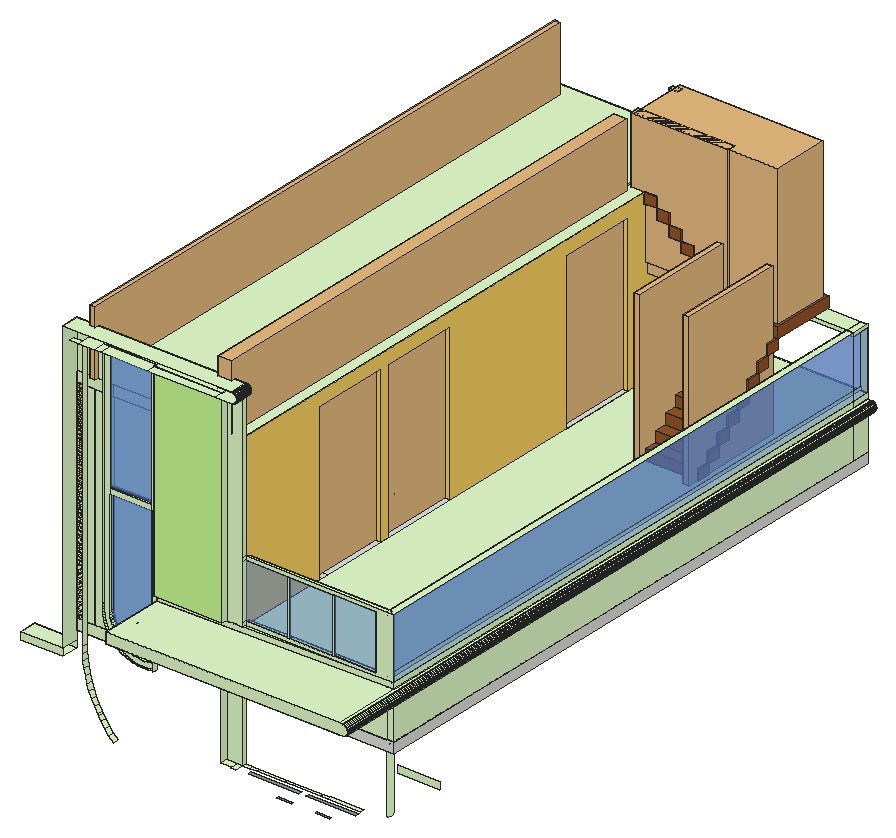
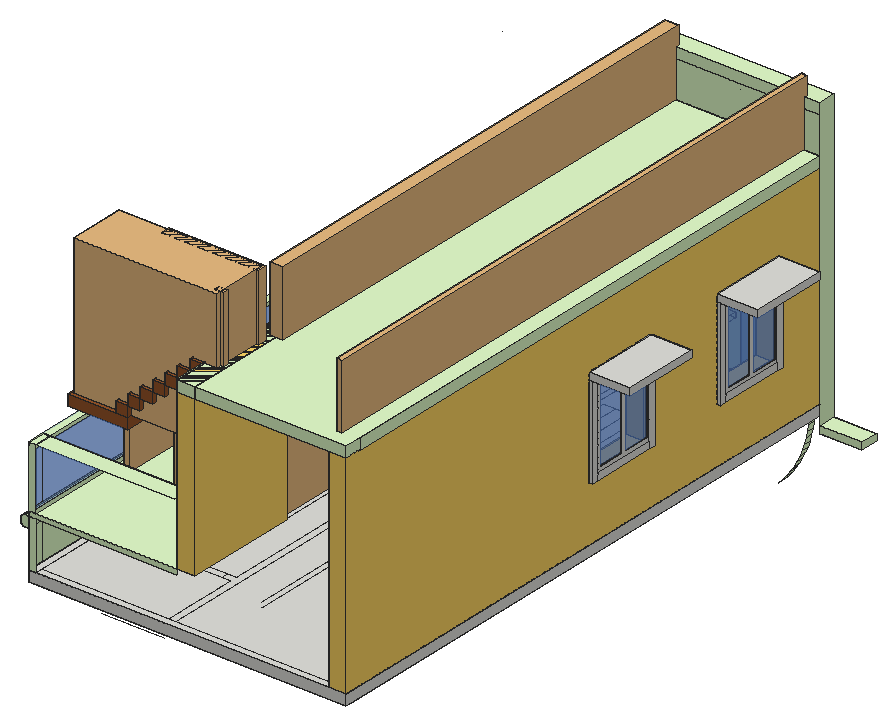
# SketchUp Ruby script. Lengths in inches.
U = 1.inch
M = Sketchup.active_model
def pt(a) = Geom::Point3d.new(a.map { |v| v * U })
def face(e, loops, mat)
  f = e.add_face(loops[0].map { |a| pt(a) })
  loops[1..].each { |l| e.add_face(l.map { |a| pt(a) }).erase! }
  f.material = f.back_material = mat if mat
  f
end
# faces: each face lists its corners as indices into pts; further lists are holes
def faces(e, pts, list, mat = nil) = list.each { |f| face(e, (f[0].is_a?(Array) ? f : [f]).map { |l| l.map { |i| pts[i] } }, mat) }
# xy, xz, yz: faces in a plane at the given z, y or x. An outline is a flat list of corners, or four numbers for a rectangle; further outlines are holes
def ring(l) = l.size == 4 ? [[l[0], l[1]], [l[2], l[1]], [l[2], l[3]], [l[0], l[3]]] : l.each_slice(2).to_a
def flat(e, list, mat, &to3) = list.each { |f| face(e, (f[0].is_a?(Array) ? f : [f]).map { |l| ring(l).map { |u, v| to3.(u, v) } }, mat) }
def xy(e, z, list, mat = nil) = flat(e, list, mat) { |x, y| [x, y, z] }
def xz(e, y, list, mat = nil) = flat(e, list, mat) { |x, z| [x, y, z] }
def yz(e, x, list, mat = nil) = flat(e, list, mat) { |y, z| [x, y, z] }
def lines(e, pts, list) = list.each { |a, b| e.add_line(pt(pts[a]), pt(pts[b])) }
# prism: a flat outline (further loops are holes) pulled along v
def prism(e, loops, v, mat = nil)
  f = face(e, loops, mat); d = Geom::Vector3d.new(v.map { |x| x * U })
  f.pushpull(f.normal.samedirection?(d) ? d.length : -d.length)
end
def box(e, o, s, mat = nil) = prism(e, [[o, [o[0] + s[0], o[1], o[2]], [o[0] + s[0], o[1] + s[1], o[2]], [o[0], o[1] + s[1], o[2]]]], [0, 0, s[2]], mat)
def at(x, y, z, deg = 0) = Geom::Transformation.translation(pt([x, y, z])) * Geom::Transformation.rotation(ORIGIN, Z_AXIS, deg.degrees)
def axes(o, x, y, z) = Geom::Transformation.new([*x, 0, *y, 0, *z, 0, *pt(o).to_a, 1])
def part(name) = M.definitions.add(name)
# library, detail: a bought-in or finely detailed component or shape, given as its bounding box
def library(name, o, s) = part(name).tap { |d| box(d.entities, o, s) }
def detail(e, o, s) = box(e.add_group.entities, o, s)
def put(e, d, t, mat = nil) = e.add_instance(d, t).tap { |i| i.material = mat if mat }
def group(e, t, mat = nil) = e.add_group.tap { |g| g.transformation = t; g.material = mat if mat }.entities
root = M.entities
M.materials.add("[Color D03]").color = [255, 216, 101]
M.materials.add("[Color F01]").color = [229, 255, 204]
M.materials.add("[Color F02]").color = [204, 255, 153]
M.materials.add("[Metal Rough]").color = [153, 157, 160]
M.materials.add("[Translucent Glass Blue]").color = [100, 149, 237]
M.materials["[Translucent Glass Blue]"].alpha = 0.5
M.materials.add("[Wood Cherry Original]").color = [152, 86, 42]
c1 = part("Difference\#3")
prism(c1.entities,[[[10,0,120],[10,0,0],[10,336,0],[10,336,120]],[[10,69,82],[10,69,36],[10,33,36],[10,33,82]],[[10,125,36],[10,125,82],[10,161,82],[10,161,36]]],[-10,0,0])
c2 = part("Group\#16")
xy(c2.entities,0,[[8.74,0,9,0,9,0.26],[140,3.98,140.02,4,140,4],[0,123.84,0.16,124,0,124],[0,335.97,0.03,336,0,336]])
p = [[145,184,0],[145,188,0],[176,288,0],[131,288,0],[176,332,0],[109,288,0],
  [104,288,0],[104,332,0],[100,188,0],[100,332,0],[104,4,0],[140,4,0],
  [4,188,0],[17,188,0],[59,188,0],[95,188,0],[4,332,0],[47,188,0],
  [176,188,0],[158,188,0],[176,284,0],[131,284,0],[104,188,0],[104,284,0],
  [109,284,0],[130.98,284,0],[109,188,0],[4,60,0],[4,96,0],[75,4,0],
  [82,4,0],[40,60,0],[40,96,0],[68,60,0],[75,60,0],[61,40,0],
  [68,40,0],[75,40,0],[82,40,0],[4,40,0],[4,47,0],[89,40,0],
  [180,0,0],[180,336,0],[4,54,0],[140,0,0],[47,96,0],[89,4,0],
  [96,4,0],[96,40,0],[61,96,0],[68,96,0],[75,96,0],[54,96,0],
  [104,0,0],[0,0,0],[0,123.84,0],[56,100,0],[56,184,0],[54,4,0],
  [61,4,0],[52,100,0],[4,100,0],[52,184,0],[47,184,0],[95,184,0],
  [47,60,0],[47,40,0],[54,40,0],[0,124,0],[0,335.97,0],[122,335.99,0],
  [122,336,0],[40,40,0],[40,47,0],[140.02,4,0],[176,4,0],[40,4,0],
  [47,4,0],[40,54,0],[8.74,0,0],[4,4,0],[104,3.33,0],[68,4,0],
  [9,0,0],[176,184,0],[0.03,336,0],[61,60,0],[54,60,0],[75,100,0],
  [59,184,0],[4,184,0],[17,184,0],[109,184,0]]
lines(c2.entities,p,[[0,1],[2,3],[4,2],[5,6],[3,5],[7,4],[6,7],[8,9],[10,11],[12,13],[14,15],[9,16],
  [13,17],[16,12],[17,14],[15,8],[18,19],[20,18],[21,20],[22,23],[23,24],[25,21],[26,22],[24,25],
  [1,26],[19,1],[27,28],[29,30],[31,32],[33,34],[35,36],[37,38],[39,40],[38,41],[42,43],[40,44],
  [45,42],[44,27],[32,46],[47,48],[30,47],[48,10],[41,49],[50,51],[51,52],[53,50],[46,53],[54,45],
  [55,56],[57,58],[59,60],[61,62],[63,64],[65,15],[31,66],[67,68],[69,70],[71,72],[73,74],[75,76],
  [77,78],[74,79],[80,55],[81,77],[73,67],[28,32],[82,10],[60,83],[84,54],[76,85],[72,86],[83,29],
  [64,17],[81,39],[61,63],[36,37],[68,35],[87,33],[66,88],[57,89],[88,87],[79,31],[52,89],[78,59],
  [88,53],[90,14],[85,0],[48,49],[30,38],[62,91],[21,3],[44,79],[72,43],[34,52],[78,67],[29,37],
  [47,41],[33,51],[59,68],[77,73],[83,36],[87,50],[90,58],[66,46],[92,13],[39,73],[24,5],[40,74],
  [60,35],[92,91],[93,26],[27,31],[93,65]])
c3 = library("Group\#21",[0,0,0],[44,4,88])
c4 = library("Group\#22",[0,0,0],[4,44,88])
c5 = library("Group\#41",[0,0,0],[3.29,59.35,85.57])
c6 = part("Group\#40")
box(c6.entities,[0,0,0],[7,36,6])
c7 = part("Group\#28")
box(c7.entities,[0,0,0],[0.5,16,22])
c8 = part("Group\#37")
yz(c8.entities,23,[[0,0,4,28],[4,0,40,4]])
p = [[23,40,28],[23,44,28],[23,40,4]]
lines(c8.entities,p,[[0,1],[0,2]])
g1 = group(c8.entities,at(23,4,0))
xz(g1,0,[[-2,0,0,4]])
g2 = group(g1,at(0,0,0))
xy(g2,0,[[-2,0,0,36]])
xy(g2,4,[[-2,0,0,36]])
xz(g2,36,[[-2,0,0,4]])
yz(g2,-2,[[0,0,36,4]])
yz(g2,0,[[0,0,36,4]])
g3 = group(c8.entities,at(23,40,0))
box(g3,[-2,0,0],[2,4,52])
g4 = group(c8.entities,at(23,0,0))
box(g4,[-2,0,0],[2,4,52])
g5 = group(c8.entities,at(22,4,4))
prism(g5,[[[0,0,0],[0,0,48],[0,36,48],[0,36,0]],[[0,35,46],[0,19,46],[0,19,2],[0,35,2]],[[0,1,2],[0,17,2],[0,17,46],[0,1,46]]],[-1,0,0])
put(g5,c7,axes([0,19,2],[-1,0,0],[0,1,0],[0,0,2]),"[Translucent Glass Blue]")
put(g5,c7,axes([-0.23,1,2],[-1,0,0],[0,1,0],[0,0,2]),"[Translucent Glass Blue]")
g6 = group(c8.entities,at(0,0,52))
yz(g6,23,[[0,0,44,4]])
g7 = group(g6,at(0,0,0))
xy(g7,0,[[0,0,23,44]])
xy(g7,4,[[0,0,23,44]])
xz(g7,0,[[0,0,23,4]])
xz(g7,44,[[0,0,23,4]])
yz(g7,0,[[0,0,44,4]])
c9 = library("Group\#42",[0,0,0],[81.24,32.15,79.17])
c10 = library("Group\#44",[0,0,0],[54.86,5.27,73.17])
c11 = library("Group\#23",[0,0,0],[3.15,329.9375,36.98])
c12 = library("Group\#43",[0,0,0],[5.02,3.15,37.57])
xy(root,75.22,[[154.51,361.07,162.66,362.07],[176.34,361.07,184.49,362.07]],"[Metal Rough]")
xy(root,82.4,[[139,360.07,167.5,362.07],[171.5,360.07,200,362.07]],"[Metal Rough]")
xy(root,85.4,[[133,355.07,136,360.07],[126.51,356.07,133,360.07],[136,360.07,139.97,362.07],[139.97,360.07,143.97,362.07],[143.97,360.07,159.98,362.07],
  [159.98,360.07,163.98,362.07],[163.98,360.07,180,362.07],[180,360.07,184,362.07],[184,360.07,203,362.07]],"[Color F01]")
xy(root,111,[[16,352.07,40,362.07]],"[Color F01]")
xy(root,115,[[16,352.07,40,362.07]],"[Color F01]")
xy(root,119.64,[[79.9,359.07,81.1875,362.07]],"[Color F01]")
xy(root,120,[[40,362.07,44,694.07],[44,362.07,216,366.07],[216,362.07,220,698.07],[40.03,694.07,216,698.07]],"[Color F01]")
xy(root,147,[[88,323.07,126.51,356.07],[126.51,323.07,136,360.07],[136,323.07,216,362.07],[216,323.07,220,362.07],[220,323.07,222,362.07],
  [220,362.07,222,698.07]],"[Color F01]")
xy(root,153,[[88,323.07,220,323.07,220,362.07,88,359.07],[220,323.07,222,698.07],[88,359.07,220,362.07,88,362.07],[216,362.07,220,698.07]],"[Color F01]")
xy(root,156,[[88,357.07,88,359.07,126.51,359.95,126.51,357.07],[88,359.07,88,362.07,126.51,362.07,126.51,359.95],[126.51,359.95,126.51,360.07,132,360.07],[126.51,360.07,126.51,362.07,136,362.07,136,360.16,132,360.07],[132,360.07,136,360.16,136,360.07],
  [136,360.16,220,362.07,216,362.07,216,364.07,136,364.07],[216,362.07,220,362.07,216,364.07],[220,362.07,220,698.07,216,698.07,216,364.07],[136,364.07,216,698.07]],"[Color F01]")
xy(root,158,[[136,362.07,159.77,364.07],[159.77,362.07,160.77,364.07],[160.77,362.07,185.55,364.07],[185.55,362.07,186.55,364.07],[186.55,362.07,210,364.07]],"[Color F01]")
xy(root,189,[[136,362.07,159.77,364.07],[159.77,362.07,160.77,364.07],[160.77,362.07,185.55,364.07],[185.55,362.07,186.55,364.07],[186.55,362.07,210,364.07]],"[Color F01]")
xy(root,191,[[136,362.07,216,364.07],[216,362.07,220,362.07,216,364.07],[220,362.07,220,688.07,216,688.07,216,364.07],[137.6,688.07,216,698.07],[216,688.07,220,698.07]],"[Color F01]")
xy(root,197.6,[[61,359.07,85,362.07]],"[Color F01]")
xy(root,200.6,[[61,359.07,85,362.07]],"[Color F01]")
xy(root,246,[[40,362.07,44,694.07],[40,694.07,40.03,698.07]],"[Color F01]")
xy(root,252,[[40,362.07,136,698.07]],"[Color F01]")
xy(root,273,[[44,352.07,49,355.07],[49,352.07,58,362.07],[58,352.07,61.61,359.07],[61.61,352.07,88,359.07],[88,352.07,126.51,357.07],
  [126.51,352.07,136,362.07],[88,357.07,88,359.07,61.61,359.07,61.61,362.07,126.51,362.07,126.51,357.07],[58,359.07,61.61,362.07]],"[Color F01]")
xy(root,279,[[40,352.07,136,362.07]],"[Color F01]")
xz(root,323.07,[[88,147,222,147,222.38,147.02,222.76,147.1,222.95,147.15,223.125,147.22,223.3,147.3,223.47,147.39,223.64,147.49,223.79,147.6,224.09,147.84,224.22,147.98,224.35,148.13,224.46,148.28,224.57,148.44,224.66,148.61,224.74,148.79,224.82,148.96,224.875,149.15,224.92,149.33,224.96,149.52,224.99,149.71,225,149.9,225,150.1,224.99,150.29,224.96,150.48,224.92,150.67,224.875,150.85,224.82,151.04,224.74,151.21,224.66,151.39,224.57,151.56,224.46,151.72,224.35,151.87,224.22,152.02,224.09,152.16,223.79,152.4,223.64,152.51,223.47,152.61,223.3,152.7,223.125,152.78,222.95,152.85,222.76,152.9,222.38,152.98,222,153,88,153]],"[Color F01]")
xz(root,352.07,[[16,111,40,115]],"[Color F01]")
xz(root,357.07,[[88,156,126.51,273]],"[Color F02]")
xz(root,359.07,[[80.83,116.63,82.29,116.69,83.75,116.85,85.18,117.1,86.6,117.45,88,117.88,88,273,61.61,273,61.61,270,85,270,85,120.13,83.74,119.89,82.47,119.72,81.1875,119.64,79.9,119.64,78.62,119.72,77.35,119.89,76.09,120.14,74.85,120.48,73.63,120.89,72.45,121.38,71.3,121.95,70.1875,122.59,69.12,123.3,68.1,124.09,67.13,124.93,66.23,125.84,65.38,126.8,64.6,127.82,63.88,128.89,63.24,130,62.67,131.15,62.17,132.33,61.76,133.55,61.61,134.08,61.42,134.79,61.17,136.05,61,137.32,61,270,61.61,270,61.61,273,58,273,58,141.42,57.91,139.96,57.91,138.5,58.01,137.04,58.2,135.59,58.49,134.16,58.87,132.75,59.33,131.36,59.89,130.01,60.53,128.7,61.25,127.43,61.61,126.88,62.06,126.21,62.94,125.04,63.9,123.9375,64.92,122.9,66.01,121.92,67.16,121.02,68.36,120.19,69.62,119.45,70.92,118.78,72.26,118.2,73.64,117.71,75.04,117.3125,76.47,117,77.92,116.78,79.37,116.66],[61,197.6,85,200.6]],"[Color F01]")
xz(root,360.07,[[126.51,85.4,136,147],[126.51,156,136,273.15]],"[Color F01]")
xz(root,362.07,[[216,87,216.29,87.05,216.58,87.11,216.87,87.2,217.14,87.3,217.42,87.42,217.68,87.5625,217.93,87.72,218.18,87.89,218.41,88.07,218.625,88.27,218.83,88.49,219.02,88.72,219.2,88.95,219.36,89.2,219.5,89.46,219.63,89.73,219.74,90.01,219.83,90.29,219.91,90.58,219.96,90.87,220,91.16,220,120,216,120],[16,111,40,115],[222,111,246,115],[79.9,119.64,81.1875,119.64,82.47,119.72,83.74,119.89,84.32,120,76.8125,120,77.35,119.89,78.62,119.72],[40,120,40,126,66.08,126,66.23,125.84,67.13,124.93,68.1,124.09,69.12,123.3,70.1875,122.59,71.3,121.95,72.45,121.38,73.63,120.89,74.85,120.48,76.09,120.14,76.8125,120],
  [84.32,120,85,120.13,85,126,136,126,136,120],[216,120,220,126],[40,126,44,246],[44,126,66.08,126,65.38,126.8,64.6,127.82,63.88,128.89,63.24,130,62.67,131.15,62.17,132.33,61.76,133.55,61.61,134.08,61.42,134.79,61.17,136.05,61,137.32,61,197.6,85,197.6,85,126,136,126,136,147,216,147,216,153,88,153,88,156,136,156,136,246,85,246,85,200.6,61,200.6,61,246,44,246],[66.08,126,85,126,85,197.6,61,197.6,61,137.32,61.17,136.05,61.42,134.79,61.61,134.08,61.76,133.55,62.17,132.33,62.67,131.15,63.24,130,63.88,128.89,64.6,127.82,65.38,126.8],
  [136,126,216,147],[216,126,220,147],[216,147,220,153],[88,153,220,153,220,191,136,191,136,189,210,189,210,158,136,158,136,156,88,156],[159.77,158,160.77,189],
  [185.55,158,186.55,189],[61,200.6,85,246],[40,246,61,252],[61,246,85,252],[85,246,136,252],
  [40,252,136,273],[40,273,40,279,136,279,136.38,278.98,136.76,278.9,136.95,278.85,137.125,278.78,137.3,278.7,137.47,278.61,137.64,278.51,137.79,278.4,138.09,278.16,138.22,278.02,138.35,277.87,138.46,277.72,138.57,277.56,138.66,277.39,138.74,277.21,138.82,277.04,138.875,276.85,138.92,276.67,138.96,276.48,138.99,276.29,139,276.1,139,275.9,138.99,275.71,138.96,275.52,138.92,275.33,138.875,275.15,138.82,274.96,138.74,274.79,138.66,274.61,138.57,274.44,138.46,274.28,138.35,274.13,138.22,273.98,138.09,273.84,137.79,273.6,137.64,273.49,137.47,273.39,137.3,273.3,137.125,273.22,136.95,273.15,136.76,273.1,136.38,273.02,136,273]],"[Color F01]")
xz(root,362.07,[[136,158,159.77,189],[160.77,158,185.55,189],[186.55,158,210,189]],"[Translucent Glass Blue]")
xz(root,364.07,[[136,156,216,158],[210,158,216,189],[136,189,216,191]],"[Color F01]")
xz(root,688.07,[[137.6,189,220,191]],"[Color F01]")
xz(root,698.07,[[216,126,220,153],[220,147,220,153,222,153,222.38,152.98,222.76,152.9,222.95,152.85,223.125,152.78,223.3,152.7,223.47,152.61,223.64,152.51,223.79,152.4,224.09,152.16,224.22,152.02,224.35,151.87,224.46,151.72,224.57,151.56,224.66,151.39,224.74,151.21,224.82,151.04,224.875,150.85,224.92,150.67,224.96,150.48,224.99,150.29,225,150.1,225,149.9,224.99,149.71,224.96,149.52,224.92,149.33,224.875,149.15,224.82,148.96,224.74,148.79,224.66,148.61,224.57,148.44,224.46,148.28,224.35,148.13,224.22,147.98,224.09,147.84,223.79,147.6,223.64,147.49,223.47,147.39,223.3,147.3,223.125,147.22,222.95,147.15,222.76,147.1,222.38,147.02,222,147],[136,153,136,156,220,156,220,153,216,153.14,216,153],[216,153,220,153,216,153.14],[216,156,220,191],
  [40,246,136,252]],"[Color F01]")
yz(root,16,[[352.07,111,362.07,115]],"[Color F01]")
yz(root,40,[[352.07,115,362.07,279],[362.07,246,688.07,252],[688.07,246,698.07,252]],"[Color F01]")
yz(root,44,[[362.07,126,366.07,246]],"[Color F01]")
yz(root,49,[[355.07,117.82,358.07,270]],"[Color F01]")
yz(root,57.91,[[358.07,138.5,359.07,139.96]],"[Color F01]")
yz(root,58,[[358.07,141.42,359.07,270]],"[Color F01]")
yz(root,61,[[359.07,137.32,362.07,197.6]],"[Color F01]")
yz(root,85,[[359.07,120.13,362.07,197.6]],"[Color F01]")
yz(root,88,[[356.07,117.88,359.07,147],[323.07,147,359.07,153],[359.07,153,362.07,156],[357.07,156,359.07,273]],"[Color F01]")
yz(root,126.51,[[356.07,85.4,360.07,147],[357.07,156,360.07,273]],"[Color F01]")
yz(root,136,[[360.07,85.4,362.07,147],[360.07,156,362.07,158],[362.07,156,364.07,158],[360.07,158,362.07,189],[360.07,189,362.07,191],
  [362.07,189,364.07,191],[360.07,191,362.07,273],[362.07,252,698.07,252.41]],"[Color F01]")
yz(root,139,[[352.07,275.9,362.07,276.1]],"[Color F01]")
yz(root,210,[[362.07,158,364.07,189]],"[Color F01]")
yz(root,216,[[364.07,156,698.07,158],[364.07,189,698.07,191]],"[Color F01]")
yz(root,216,[[364.07,158,698.07,189]],"[Translucent Glass Blue]")
yz(root,220,[[362.07,126,688.07,147],[688.07,126,698.07,147],[362.07,147,688.07,153],[688.07,147,698.07,153],[362.07,153,688.07,156],
  [688.07,153,698.07,156],[688.07,189,698.07,191]],"[Color F01]")
yz(root,220,[[362.07,156,688.07,191],[688.07,156,698.07,189]],"[Translucent Glass Blue]")
yz(root,225,[[323.07,149.9,698.07,150.1]],"[Color F01]")
p = [[66.49,358.07,75.01],[63.97,358.07,77.66],[63.97,355.07,77.66],[66.49,355.07,75.01],[61.61,358.07,80.45],[61.61,355.07,80.45],
  [59.44,358.07,83.39],[59.44,355.07,83.39],[58.14,358.07,85.4],[58.14,355.07,85.4],[57.45,358.07,86.46],[57.45,355.07,86.46],
  [55.66,358.07,89.65],[55.66,355.07,89.65],[54.07,358.07,92.9375],[54.07,355.07,92.9375],[52.6875,358.07,96.32],[52.6875,355.07,96.32],
  [51.52,358.07,99.79],[51.52,355.07,99.79],[50.57,358.07,103.32],[50.57,355.07,103.32],[49.84,358.07,106.9],[49.84,355.07,106.9],
  [49.33,358.07,110.52],[49.33,355.07,110.52],[49.05,358.07,114.16],[49.05,355.07,114.16],[49,358.07,117.82],[49,355.07,117.82],
  [80.83,358.07,116.63],[80.83,359.07,116.63],[79.37,359.07,116.66],[79.37,358.07,116.66],[82.29,358.07,116.69],[82.29,359.07,116.69],
  [77.92,359.07,116.78],[77.92,358.07,116.78],[83.75,358.07,116.85],[83.75,359.07,116.85],[76.47,359.07,117],[76.47,358.07,117],
  [85.18,358.07,117.1],[85.18,359.07,117.1],[75.04,359.07,117.3125],[75.04,358.07,117.3125],[86.6,358.07,117.45],[86.6,359.07,117.45],
  [73.64,359.07,117.71],[73.64,358.07,117.71],[88,358.07,117.88],[88,359.07,117.88],[72.26,359.07,118.2],[72.26,358.07,118.2],
  [70.92,359.07,118.78],[70.92,358.07,118.78],[69.62,359.07,119.45],[69.62,358.07,119.45],[68.36,359.07,120.19],[68.36,358.07,120.19],
  [78.62,359.07,119.72],[79.9,359.07,119.64],[79.9,362.07,119.64],[78.62,362.07,119.72],[81.1875,359.07,119.64],[82.47,359.07,119.72],
  [82.47,362.07,119.72],[81.1875,362.07,119.64],[77.35,359.07,119.89],[77.35,362.07,119.89],[83.74,359.07,119.89],[83.74,362.07,119.89],
  [76.09,359.07,120.14],[76.8125,362.07,120],[76.09,362.07,120.14],[85,359.07,120.13],[85,362.07,120.13],[84.32,362.07,120],
  [74.85,359.07,120.48],[74.85,362.07,120.48],[67.16,359.07,121.02],[67.16,358.07,121.02],[73.63,359.07,120.89],[73.63,362.07,120.89],
  [72.45,359.07,121.38],[72.45,362.07,121.38],[66.01,359.07,121.92],[66.01,358.07,121.92],[71.3,359.07,121.95],[71.3,362.07,121.95],
  [64.92,359.07,122.9],[64.92,358.07,122.9],[70.1875,359.07,122.59],[70.1875,362.07,122.59],[69.12,359.07,123.3],[69.12,362.07,123.3],
  [63.9,359.07,123.9375],[63.9,358.07,123.9375],[68.1,359.07,124.09],[68.1,362.07,124.09],[62.94,359.07,125.04],[62.94,358.07,125.04],
  [67.13,359.07,124.93],[67.13,362.07,124.93],[66.23,359.07,125.84],[66.23,362.07,125.84],[62.06,359.07,126.21],[62.06,358.07,126.21],
  [65.38,359.07,126.8],[66.08,362.07,126],[65.38,362.07,126.8],[61.61,359.07,126.88],[61.61,358.07,126.88],[64.6,359.07,127.82],
  [64.6,362.07,127.82],[61.25,359.07,127.43],[61.25,358.07,127.43],[60.53,359.07,128.7],[60.53,358.07,128.7],[63.88,359.07,128.89],
  [63.88,362.07,128.89],[59.89,359.07,130.01],[59.89,358.07,130.01],[63.24,359.07,130],[63.24,362.07,130],[59.33,359.07,131.36],
  [59.33,358.07,131.36],[62.67,359.07,131.15],[62.67,362.07,131.15],[62.17,359.07,132.33],[62.17,362.07,132.33],[58.87,359.07,132.75],
  [58.87,358.07,132.75],[61.76,359.07,133.55],[61.76,362.07,133.55],[58.49,359.07,134.16],[58.49,358.07,134.16],[61.61,359.07,134.08],
  [61.61,362.07,134.08],[61.42,359.07,134.79],[61.42,362.07,134.79],[58.2,359.07,135.59],[58.2,358.07,135.59],[61.17,359.07,136.05],
  [61.17,362.07,136.05],[58.01,359.07,137.04],[58.01,358.07,137.04],[61,359.07,137.32],[61,362.07,137.32],[57.91,359.07,138.5],
  [57.91,358.07,138.5],[57.91,358.07,139.96],[57.91,359.07,139.96],[58,359.07,141.42],[58,358.07,141.42],[222,323.07,147],
  [222,362.07,147],[222,698.07,147],[222.19,698.07,147.01],[222.19,323.07,147.01],[222.38,698.07,147.02],[222.38,323.07,147.02],
  [222.57,698.07,147.06],[222.57,323.07,147.06],[222.76,698.07,147.1],[222.76,323.07,147.1],[222.95,698.07,147.15],[222.95,323.07,147.15],
  [223.125,698.07,147.22],[223.125,323.07,147.22],[223.3,698.07,147.3],[223.3,323.07,147.3],[223.47,698.07,147.39],[223.47,323.07,147.39],
  [223.64,698.07,147.49],[223.64,323.07,147.49],[223.79,698.07,147.6],[223.79,323.07,147.6],[223.94,698.07,147.72],[223.94,323.07,147.72],
  [224.09,698.07,147.84],[224.09,323.07,147.84],[224.22,698.07,147.98],[224.22,323.07,147.98],[224.35,698.07,148.13],[224.35,323.07,148.13],
  [224.46,698.07,148.28],[224.46,323.07,148.28],[224.57,698.07,148.44],[224.57,323.07,148.44],[224.66,698.07,148.61],[224.66,323.07,148.61],
  [224.74,698.07,148.79],[224.74,323.07,148.79],[224.82,698.07,148.96],[224.82,323.07,148.96],[224.875,698.07,149.15],[224.875,323.07,149.15],
  [224.92,698.07,149.33],[224.92,323.07,149.33],[224.96,698.07,149.52],[224.96,323.07,149.52],[224.99,698.07,149.71],[224.99,323.07,149.71],
  [225,698.07,149.9],[225,323.07,149.9],[225,323.07,150.1],[225,698.07,150.1],[224.99,698.07,150.29],[224.99,323.07,150.29],
  [224.96,698.07,150.48],[224.96,323.07,150.48],[224.92,698.07,150.67],[224.92,323.07,150.67],[224.875,698.07,150.85],[224.875,323.07,150.85],
  [224.82,698.07,151.04],[224.82,323.07,151.04],[224.74,698.07,151.21],[224.74,323.07,151.21],[224.66,698.07,151.39],[224.66,323.07,151.39],
  [224.57,698.07,151.56],[224.57,323.07,151.56],[224.46,698.07,151.72],[224.46,323.07,151.72],[224.35,698.07,151.87],[224.35,323.07,151.87],
  [224.22,698.07,152.02],[224.22,323.07,152.02],[224.09,698.07,152.16],[224.09,323.07,152.16],[223.94,698.07,152.28],[223.94,323.07,152.28],
  [223.79,698.07,152.4],[223.79,323.07,152.4],[223.64,698.07,152.51],[223.64,323.07,152.51],[223.47,698.07,152.61],[223.47,323.07,152.61],
  [223.3,698.07,152.7],[223.3,323.07,152.7],[223.125,698.07,152.78],[223.125,323.07,152.78],[222.95,323.07,152.85],[222.95,698.07,152.85],
  [222.76,698.07,152.9],[222.76,323.07,152.9],[222.57,323.07,152.94],[222.57,698.07,152.94],[222.38,698.07,152.98],[222.38,323.07,152.98],
  [222.19,323.07,152.99],[222.19,698.07,152.99],[222,698.07,153],[222,323.07,153],[220,362.07,153],[220,362.07,156],
  [136,360.16,156],[132,360.07,156],[126.51,359.95,156],[88,359.07,156],[88,359.07,153],[220,362.07,191],
  [216,364.07,191],[216,364.07,189],[216,364.07,158],[216,364.07,156],[136,362.07,273],[136.19,362.07,273.01],
  [136.19,352.07,273.01],[136,352.07,273],[136,360.07,273],[136.38,362.07,273.02],[136.38,352.07,273.02],[136.57,362.07,273.06],
  [136.57,352.07,273.06],[136.76,362.07,273.1],[136.76,352.07,273.1],[136.95,362.07,273.15],[136.95,352.07,273.15],[137.125,362.07,273.22],
  [137.125,352.07,273.22],[137.3,362.07,273.3],[137.3,352.07,273.3],[137.47,362.07,273.39],[137.47,352.07,273.39],[137.64,362.07,273.49],
  [137.64,352.07,273.49],[137.79,362.07,273.6],[137.79,352.07,273.6],[137.94,362.07,273.72],[137.94,352.07,273.72],[138.09,362.07,273.84],
  [138.09,352.07,273.84],[138.22,362.07,273.98],[138.22,352.07,273.98],[138.35,362.07,274.13],[138.35,352.07,274.13],[138.46,362.07,274.28],
  [138.46,352.07,274.28],[138.57,362.07,274.44],[138.57,352.07,274.44],[138.66,362.07,274.61],[138.66,352.07,274.61],[138.74,362.07,274.79],
  [138.74,352.07,274.79],[138.82,362.07,274.96],[138.82,352.07,274.96],[138.875,362.07,275.15],[138.875,352.07,275.15],[138.92,362.07,275.33],
  [138.92,352.07,275.33],[138.96,362.07,275.52],[138.96,352.07,275.52],[138.99,362.07,275.71],[138.99,352.07,275.71],[139,362.07,275.9],
  [139,352.07,275.9],[139,362.07,276.1],[138.99,362.07,276.29],[138.99,352.07,276.29],[139,352.07,276.1],[138.96,362.07,276.48],
  [138.96,352.07,276.48],[138.92,362.07,276.67],[138.92,352.07,276.67],[138.875,362.07,276.85],[138.875,352.07,276.85],[138.82,362.07,277.04],
  [138.82,352.07,277.04],[138.74,362.07,277.21],[138.74,352.07,277.21],[138.66,362.07,277.39],[138.66,352.07,277.39],[138.57,362.07,277.56],
  [138.57,352.07,277.56],[138.46,362.07,277.72],[138.46,352.07,277.72],[138.35,362.07,277.87],[138.35,352.07,277.87],[138.22,362.07,278.02],
  [138.22,352.07,278.02],[138.09,362.07,278.16],[138.09,352.07,278.16],[137.94,362.07,278.28],[137.94,352.07,278.28],[137.79,362.07,278.4],
  [137.79,352.07,278.4],[137.64,362.07,278.51],[137.64,352.07,278.51],[137.47,362.07,278.61],[137.47,352.07,278.61],[137.3,362.07,278.7],
  [137.3,352.07,278.7],[137.125,362.07,278.78],[137.125,352.07,278.78],[136.95,362.07,278.85],[136.76,362.07,278.9],[136.76,352.07,278.9],
  [136.95,352.07,278.85],[136.57,362.07,278.94],[136.38,362.07,278.98],[136.38,352.07,278.98],[136.57,352.07,278.94],[136.19,362.07,278.99],
  [136,362.07,279],[136,352.07,279],[136.19,352.07,278.99],[136,284.07,191],[136,286.07,191],[220,362.07,252.41],
  [220,362.07,252],[180,441.07,91.09],[144,441.07,91.09],[180,437.07,91.09],[144,437.07,91.09],[136,698.07,246],
  [136,698.07,156],[40.03,698.07,126],[40.03,694.07,126],[44,366.07,126],[44,694.07,126],[216,698.07,126],
  [40,694.07,126],[40,688.07,126],[216,694.07,126],[61,362.07,270],[61,359.07,270],[85,362.07,270],
  [85,359.07,270],[126.51,362.07,273.15],[126.51,360.07,273.15],[136,362.07,273.15],[136,360.07,273.15],[216,362.07,158],
  [216,362.07,189],[216,366.07,126],[88,362.07,153],[88,698.07,153],[88,362.07,156],[88,698.07,156],
  [126.51,362.07,156],[126.51,698.07,156],[187.19,688.07,111],[151.19,688.07,111],[40,362.07,126],[50.5,362.07,252],
  [50.5,688.07,252]]
faces(root,p,[[0,1,2,3],[1,4,5,2],[4,6,7,5],[6,8,9,7],[8,10,11,9],[10,12,13,11],[12,14,15,13],[14,16,17,15],
  [16,18,19,17],[18,20,21,19],[20,22,23,21],[22,24,25,23],[24,26,27,25],[26,28,29,27],[30,31,32,33],[34,35,31,30],
  [33,32,36,37],[38,39,35,34],[37,36,40,41],[42,43,39,38],[41,40,44,45],[46,47,43,42],[45,44,48,49],[50,51,47,46],
  [49,48,52,53],[53,52,54,55],[55,54,56,57],[57,56,58,59],[60,61,62,63],[64,65,66,67],[68,60,63,69],[65,70,71,66],
  [72,68,69,73,74],[70,75,76,77,71],[78,72,74,79],[59,58,80,81],[82,78,79,83],[84,82,83,85],[81,80,86,87],[88,84,85,89],
  [87,86,90,91],[92,88,89,93],[94,92,93,95],[91,90,96,97],[98,94,95,99],[97,96,100,101],[102,98,99,103],[104,102,103,105],
  [101,100,106,107],[108,104,105,109,110],[107,106,111,112],[113,108,110,114],[112,111,115,116],[116,115,117,118],[119,113,114,120],[118,117,121,122],
  [123,119,120,124],[122,121,125,126],[127,123,124,128],[129,127,128,130],[126,125,131,132],[133,129,130,134],[132,131,135,136],[137,133,134,138],
  [139,137,138,140],[136,135,141,142],[143,139,140,144],[142,141,145,146],[147,143,144,148],[146,145,149,150],[151,152,153,154],[155,156,157,158,159],
  [159,158,160,161],[161,160,162,163],[163,162,164,165],[165,164,166,167],[167,166,168,169],[169,168,170,171],[171,170,172,173],[173,172,174,175],
  [175,174,176,177],[177,176,178,179],[179,178,180,181],[181,180,182,183],[183,182,184,185],[185,184,186,187],[187,186,188,189],[189,188,190,191],
  [191,190,192,193],[193,192,194,195],[195,194,196,197],[197,196,198,199],[199,198,200,201],[201,200,202,203],[203,202,204,205],[206,207,208,209],
  [209,208,210,211],[211,210,212,213],[213,212,214,215],[215,214,216,217],[217,216,218,219],[219,218,220,221],[221,220,222,223],[223,222,224,225],
  [225,224,226,227],[227,226,228,229],[229,228,230,231],[231,230,232,233],[233,232,234,235],[235,234,236,237],[237,236,238,239],[239,238,240,241],
  [241,240,242,243],[244,245,246,247],[243,242,245,244],[248,249,250,251],[247,246,249,248],[252,253,254,255],[251,250,253,252],[256,257,258,259,260,261,262],
  [263,264,265,266,267,257],[268,269,270,271,272],[269,273,274,270],[273,275,276,274],[275,277,278,276],[277,279,280,278],[279,281,282,280],[281,283,284,282],
  [283,285,286,284],[285,287,288,286],[287,289,290,288],[289,291,292,290],[291,293,294,292],[293,295,296,294],[295,297,298,296],[297,299,300,298],
  [299,301,302,300],[301,303,304,302],[303,305,306,304],[305,307,308,306],[307,309,310,308],[309,311,312,310],[311,313,314,312],[313,315,316,314],
  [315,317,318,316],[319,320,321,322],[320,323,324,321],[323,325,326,324],[325,327,328,326],[327,329,330,328],[329,331,332,330],[331,333,334,332],
  [333,335,336,334],[335,337,338,336],[337,339,340,338],[339,341,342,340],[341,343,344,342],[343,345,346,344],[345,347,348,346],[347,349,350,348],
  [349,351,352,350],[351,353,354,352],[353,355,356,354],[357,358,359,360],[355,357,360,356],[361,362,363,364],[358,361,364,359],[365,366,367,368],
  [362,365,368,363]],"[Color F01]")
lines(root,p,[[369,370],[371,372],[373,374],[375,376],[377,378],[379,380],[381,382],[383,379],[380,384],[384,385],[382,380],[383,386],
  [382,386],[387,388],[389,390],[391,392],[393,394],[395,266],[396,265],[397,381],[386,397],[398,399],[400,401],[402,403],
  [404,405],[385,406],[407,408]])
g8 = group(root,at(61,362.07,119.64),"[Translucent Glass Blue]")
prism(g8,[[[0,-1,77.96],[0,-1,17.68],[0.17,-1,16.41],[0.42,-1,15.15],[0.61,-1,14.44],[0.76,-1,13.91],[1.17,-1,12.7],[1.67,-1,11.51],[2.24,-1,10.36],[2.88,-1,9.25],[3.6,-1,8.18],[4.38,-1,7.16],[5.23,-1,6.2],[6.13,-1,5.29],[7.1,-1,4.45],[8.12,-1,3.67],[9.1875,-1,2.95],[10.3,-1,2.3125],[11.45,-1,1.74],[12.63,-1,1.25],[13.85,-1,0.84],[15.09,-1,0.51],[16.35,-1,0.26],[17.62,-1,0.09],[18.9,-1,0],[20.1875,-1,0],[21.47,-1,0.08],[22.74,-1,0.25],[24,-1,0.5],[24,-1,77.96]]],[0,1,0])
g9 = group(root,at(40,362.07,120))
box(g9,[0,0,0],[180,336,6])
put(root,c1,at(40,362.07,126),"[Color D03]")
put(root,c2,at(40,362.07,126))
g10 = group(root,at(126,362.07,156),"[Color D03]")
xy(g10,0,[[0,0,10,52],[3,52,7,56],[3,92,7,96],[0,96,10,101],[0,145,10,227],
  [0,271,10,336]])
xy(g10,88,[[0,52,10,96],[0,101,10,145],[0,227,10,271]])
xy(g10,96,[[0,0,10,336]])
xz(g10,0,[[0,0,10,96]])
xz(g10,52,[[0,0,10,88]])
xz(g10,96,[[0,0,10,88]])
xz(g10,101,[[0,0,10,88]])
xz(g10,145,[[0,0,10,88]])
xz(g10,227,[[0,0,10,88]])
xz(g10,271,[[0,0,10,88]])
xz(g10,336,[[0,0,10,96]])
yz(g10,0,[[0,0,0,96,336,96,336,0,271,0,271,88,227,88,227,0,145,0,145,88,101,88,101,0,96,0,96,88,52,88,52,0]])
yz(g10,10,[[0,0,52,0,52,88,96,88,96,0,101,0,101,88,145,88,145,0,227,0,227,88,271,88,271,0,336,0,336,96,0,96]])
p = [[10,271,0],[10,227,0]]
lines(g10,p,[[0,1]])
put(g10,c3,at(7,52,0,90))
put(g10,c4,at(3,227,0))
put(g10,c4,at(3,100.9375,0))
put(root,c5,at(207.125,583.28,156))
put(root,c6,at(176,595.62,156.41,-90),"[Wood Cherry Original]")
put(root,c5,at(177.92,584.74,156.41))
put(root,c8,at(17,481.9,158))
put(root,c8,at(17,391.11,158))
put(root,c6,at(176,602.62,162.41,-90),"[Wood Cherry Original]")
put(root,c6,at(176,609.62,168.41,-90),"[Wood Cherry Original]")
put(root,c6,at(176,616.62,174.41,-90),"[Wood Cherry Original]")
put(root,c6,at(176,623.62,180.41,-90),"[Wood Cherry Original]")
put(root,c6,at(176,630.62,186.41,-90),"[Wood Cherry Original]")
put(root,c6,at(176,637.62,192.41,-90),"[Wood Cherry Original]")
put(root,c6,at(176,644.62,198.41,-90),"[Wood Cherry Original]")
g11 = group(root,at(61.02,360.98,200.6),"[Translucent Glass Blue]")
box(g11,[0,-1,0],[24,1,69.4])
g12 = group(root,at(185,644.62,204.41),"[Wood Cherry Original]")
box(g12,[-7,0,0],[34,36,6])
put(root,c6,at(178,644.62,210.41),"[Wood Cherry Original]")
put(root,c9,at(129.29,646.21,210.41))
put(root,c6,at(171,644.62,216.41),"[Wood Cherry Original]")
put(root,c10,at(127.93,645.19,216.41))
put(root,c6,at(164,644.62,222.41),"[Wood Cherry Original]")
put(root,c6,at(157,644.62,228.41),"[Wood Cherry Original]")
put(root,c6,at(150,644.62,234.41),"[Wood Cherry Original]")
put(root,c6,at(143,644.62,240.41),"[Wood Cherry Original]")
put(root,c6,at(136,644.62,246.41),"[Wood Cherry Original]")
put(root,c11,at(48.93,360.1,252))
put(root,c12,at(127.43,672.7,252))
put(root,c11,axes([121.875,360.1,252],[2.39,0,0],[0,0.85,0],[0,0,1]))
